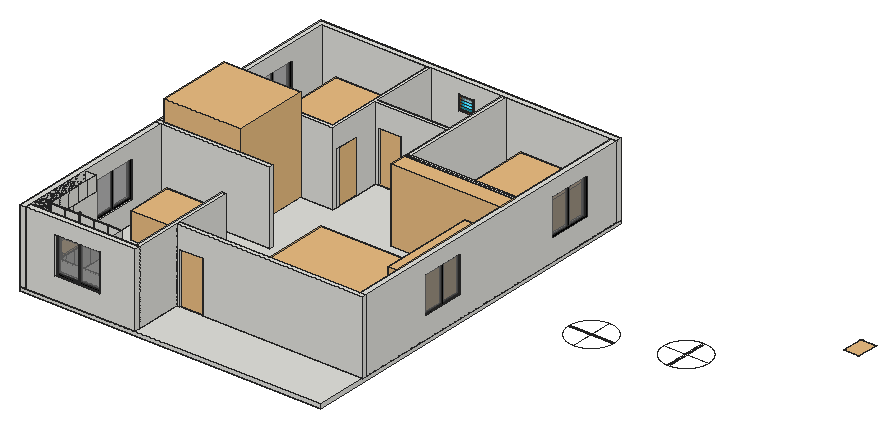
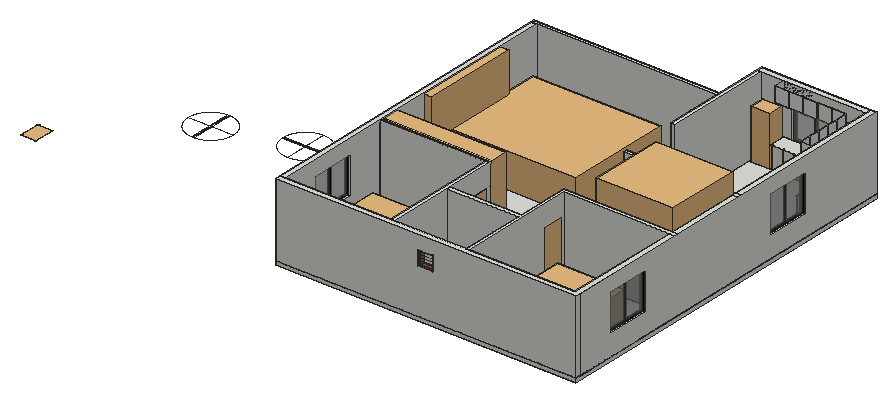
# SketchUp Ruby script. Lengths in inches.
U = 1.inch
M = Sketchup.active_model
def pt(a) = Geom::Point3d.new(a.map { |v| v * U })
def face(e, loops, mat)
  f = e.add_face(loops[0].map { |a| pt(a) })
  loops[1..].each { |l| e.add_face(l.map { |a| pt(a) }).erase! }
  f.material = f.back_material = mat if mat
  f
end
# faces: each face lists its corners as indices into pts; further lists are holes
def faces(e, pts, list, mat = nil) = list.each { |f| face(e, (f[0].is_a?(Array) ? f : [f]).map { |l| l.map { |i| pts[i] } }, mat) }
# xy, xz, yz: faces in a plane at the given z, y or x. An outline is a flat list of corners, or four numbers for a rectangle; further outlines are holes
def ring(l) = l.size == 4 ? [[l[0], l[1]], [l[2], l[1]], [l[2], l[3]], [l[0], l[3]]] : l.each_slice(2).to_a
def flat(e, list, mat, &to3) = list.each { |f| face(e, (f[0].is_a?(Array) ? f : [f]).map { |l| ring(l).map { |u, v| to3.(u, v) } }, mat) }
def xy(e, z, list, mat = nil) = flat(e, list, mat) { |x, y| [x, y, z] }
def xz(e, y, list, mat = nil) = flat(e, list, mat) { |x, z| [x, y, z] }
def yz(e, x, list, mat = nil) = flat(e, list, mat) { |y, z| [x, y, z] }
def lines(e, pts, list) = list.each { |a, b| e.add_line(pt(pts[a]), pt(pts[b])) }
# prism: a flat outline (further loops are holes) pulled along v
def prism(e, loops, v, mat = nil)
  f = face(e, loops, mat); d = Geom::Vector3d.new(v.map { |x| x * U })
  f.pushpull(f.normal.samedirection?(d) ? d.length : -d.length)
end
def box(e, o, s, mat = nil) = prism(e, [[o, [o[0] + s[0], o[1], o[2]], [o[0] + s[0], o[1] + s[1], o[2]], [o[0], o[1] + s[1], o[2]]]], [0, 0, s[2]], mat)
def at(x, y, z, deg = 0) = Geom::Transformation.translation(pt([x, y, z])) * Geom::Transformation.rotation(ORIGIN, Z_AXIS, deg.degrees)
def axes(o, x, y, z) = Geom::Transformation.new([*x, 0, *y, 0, *z, 0, *pt(o).to_a, 1])
def part(name) = M.definitions.add(name)
# library, detail: a bought-in or finely detailed component or shape, given as its bounding box
def library(name, o, s) = part(name).tap { |d| box(d.entities, o, s) }
def detail(e, o, s) = box(e.add_group.entities, o, s)
def put(e, d, t, mat = nil) = e.add_instance(d, t).tap { |i| i.material = mat if mat }
def group(e, t, mat = nil) = e.add_group.tap { |g| g.transformation = t; g.material = mat if mat }.entities
root = M.entities
M.materials.add("[Color_008]").color = [30, 30, 30]
M.materials.add("[Color_009]").color = [0, 0, 0]
M.materials.add("[Translucent Glass Gray]").color = [128, 128, 128]
M.materials["[Translucent Glass Gray]"].alpha = 0.5
M.materials.add("[Translucent Glass Tinted]1").color = [7, 201, 240]
M.materials["[Translucent Glass Tinted]1"].alpha = 0.48
M.materials.add("[Translucent_Glass_Gray]").color = [128, 128, 128]
M.materials["[Translucent_Glass_Gray]"].alpha = 0.5
M.materials.add("[Wood Cherry Original]").color = [152, 86, 42]
M.materials.add("[Wood Floor Parquet]").color = [145, 89, 39]
c1 = library("bed",[-25.65,-58.99,0],[75.48,89.46,37.24])
c2 = library("sofa+(2)",[-100.93,-81.02,-0.06],[174.43,145.32,46.54])
c3 = library("DINING+TABLE_4+SEATER_+1200mm+x+900mm",[14.07,13.24,0],[72.26,62.1,36.02])
c4 = library("main+door",[0,-0.79,0],[47.24,7.88,82.68])
c5 = part("ventilator")
g1 = group(c5.entities,at(0,0,0))
xy(g1,0,[[0,0,24,1],[0,1,24,6.83]],"[Wood Floor Parquet]")
xy(g1,1.75,[[2,0,22,6.83]],"[Wood Floor Parquet]")
xy(g1,21.87,[[2,0,22,6.83]],"[Wood Cherry Original]")
xy(g1,23.62,[[0,0,24,1],[0,1,24,6.83]],"[Wood Floor Parquet]")
xz(g1,0,[[[0,0,24,23.62],[2,1.75,22,21.87]]],"[Wood Floor Parquet]")
xz(g1,6.83,[[[0,0,24,23.62],[2,1.75,22,21.87]]],"[Wood Cherry Original]")
yz(g1,0,[[0,0,1,23.62],[1,0,6.83,23.62]],"[Wood Floor Parquet]")
yz(g1,2,[[0,1.75,6.83,1.75,6.83,7.66,0,3.5],[0,3.5,6.83,7.66,6.83,11.8125,0,7.66],[0,7.66,6.83,11.8125,6.83,15.97,0,11.8125],[0,11.8125,6.83,15.97,6.83,20.12,0,15.97],[0,15.97,6.83,20.12,6.83,21.87,0,21.87]],"[Wood Floor Parquet]")
yz(g1,22,[[0,1.75,0,3.5,6.83,7.66,6.83,1.75],[0,3.5,0,7.66,6.83,11.8125,6.83,7.66],[0,7.66,0,11.8125,6.83,15.97,6.83,11.8125],[0,11.8125,0,15.97,6.83,20.12,6.83,15.97],[0,15.97,0,21.87,6.83,21.87,6.83,20.12]],"[Wood Floor Parquet]")
yz(g1,24,[[0,0,1,23.62],[1,0,6.83,23.62]],"[Wood Floor Parquet]")
p = [[2,0,3.5],[2,6.83,7.66],[22,6.83,7.66],[22,0,3.5],[2,6.83,11.8125],[2,0,7.66],
  [22,0,7.66],[22,6.83,11.8125],[2,0,11.8125],[2,6.83,15.97],[22,6.83,15.97],[22,0,11.8125],
  [2,6.83,20.12],[2,0,15.97],[22,0,15.97],[22,6.83,20.12]]
faces(g1,p,[[0,1,2,3],[4,5,6,7],[8,9,10,11]],"[Translucent Glass Tinted]1")
faces(g1,p,[[12,13,14,15]],"[Translucent Glass Gray]")
c6 = part("Group\#2")
xy(c6.entities,0,[[0,0,82.68,1.18]],"[Color_009]")
xy(c6.entities,1.97,[[1.97,0.98,40.35,1.18],[42.32,0.98,80.71,1.18]])
xy(c6.entities,1.97,[[1.97,0,40.35,0.3],[42.32,0,80.71,0.3]],"[Color_009]")
xy(c6.entities,80.71,[[1.97,0,40.35,0.3],[42.32,0,80.71,0.3],[1.97,0.3,40.35,0.98],[42.32,0.3,80.71,0.98],[1.97,0.98,40.35,1.18],
  [42.32,0.98,80.71,1.18]])
xy(c6.entities,82.68,[[0,0,82.68,1.18]],"[Color_008]")
xz(c6.entities,0,[[[0,0,82.68,82.68],[1.97,1.97,40.35,80.71],[42.32,1.97,80.71,80.71]]],"[Color_009]")
xz(c6.entities,0.3,[[1.97,1.97,40.35,80.71],[42.32,1.97,80.71,80.71]],"[Translucent_Glass_Gray]")
xz(c6.entities,0.98,[[1.97,1.97,40.35,80.71],[42.32,1.97,80.71,80.71]],"[Translucent_Glass_Gray]")
xz(c6.entities,1.18,[[[0,0,82.68,82.68],[1.97,1.97,80.71,80.71]],[40.35,1.97,42.32,80.71]],"[Color_009]")
yz(c6.entities,0,[[0,0,1.18,82.68]],"[Color_009]")
yz(c6.entities,1.97,[[0.98,1.97,1.18,80.71]])
yz(c6.entities,1.97,[[0,1.97,0.3,80.71]],"[Color_009]")
yz(c6.entities,40.35,[[0,1.97,0.3,80.71],[0.98,1.97,1.18,80.71]],"[Color_009]")
yz(c6.entities,42.32,[[0,1.97,0.3,80.71],[0.98,1.97,1.18,80.71]])
yz(c6.entities,80.71,[[0,1.97,0.3,80.71],[0.98,1.97,1.18,80.71]],"[Color_009]")
yz(c6.entities,82.68,[[0,0,1.18,82.68]],"[Color_009]")
c7 = library("A$C150B42AD",[-2.96,-4.03,0],[5.92,8.06,0.01])
c8 = library("Component\#33",[0,0,0],[60.64,55.48,158.625])
c9 = library("CS300DRT",[0,0,0],[27.18,17.85,30.31])
c10 = library("Group\#6",[0,0,0],[122,120,150.6])
c11 = library("Group\#13",[0,-2.07,0],[175.11,29.89,117.3125])
c12 = library("Curtain set",[2.63,-1.46,0.02],[153.32,14.02,114.15])
c13 = library("Gas range top",[0,0,34.52],[24.41,48.07,2.63])
c14 = library("SKT_Nearly Natural 5' Kentia Palm Silk Tree",[-23.18,-17.61,0],[47.48,43.95,59.125])
c15 = part("Inclined chimney")
g2 = group(c15.entities,at(1.97,2.08,2.89))
xy(g2,0,[[0,7.9,31.3,13.68]])
xy(g2,11.29,[[0,0,31.3,13.68]])
xz(g2,13.68,[[0,0,31.3,11.29]])
yz(g2,0,[[7.9,0,0,11.29,13.68,11.29,13.68,0]])
yz(g2,31.3,[[7.9,0,13.68,0,13.68,11.29,0,11.29]])
g3 = group(c15.entities,at(0,9.85,0.4))
g4 = group(g3,at(0,0.61,0.43))
prism(g4,[[[35.24,0,0],[35.24,-3.39,4.84],[35.24,-3.58,4.7],[35.24,-0.29,0]]],[-35.24,0,0])
g5 = group(g3,at(0,-3.21,4.99))
prism(g5,[[[35.24,-0.2,-0.12],[35.24,-3.16,5],[0,-3.16,5],[0,-0.2,-0.12]]],[0,0.2,0.12])
g6 = group(g3,at(0,-6.27,10.27))
prism(g6,[[[35.24,-0.19,-0.14],[35.24,-3.58,4.7],[0,-3.58,4.7],[0,-0.19,-0.14]]],[0,0.19,0.14])
g7 = group(g3,at(0,0.61,0.43))
prism(g7,[[[35.24,0,0],[35.24,0.96,0],[35.24,-9.52,14.96],[35.24,-10.16,14.51]]],[-35.24,0,0])
g8 = group(c15.entities,at(10.24,3.95,20.8))
box(g8,[0,0,-6.62],[14.76,11.8125,20.56])
g9 = group(c15.entities,at(0,10.1,0))
prism(g9,[[[35.24,0.46,0],[35.24,1.33,0],[35.24,1.33,0.83],[35.24,1.01,0.83],[35.24,0.37,0.83],[35.24,0,0.83],[35.24,0,0.64]]],[-35.24,0,0])
c16 = part("Inclined+chimney")
put(c16.entities,c15,at(34.17,38.97,0.69))
xy(root,0,[[259.625,9,283.625,32.9],[259.625,32.9,283.625,104.9]])
xy(root,0.2,[[283.82,32.9,301.42,33.08],[301.82,32.9,319.42,33.08],[319.82,32.9,355.42,33.08],[355.82,32.9,373.42,33.08],[373.82,32.9,391.42,33.08],
  [283.625,33.1,283.8,49.49],[283.625,49.89,283.8,66.28],[283.625,66.68,283.8,80.9],[283.625,80.9,283.8,83.07],[283.625,83.47,283.8,99.85],
  [283.625,100.25,283.8,104.9],[283.625,104.9,283.8,116.64]])
xy(root,11.8,[[319.82,32.9,355.42,33.08]])
xy(root,12.2,[[319.82,32.9,355.42,33.08]])
xy(root,23.8,[[319.82,32.9,355.42,33.08]])
xy(root,24.2,[[319.82,32.9,355.42,33.08]])
xy(root,35.8,[[283.82,32.9,301.42,33.08],[301.82,32.9,319.42,33.08],[319.82,32.9,355.42,33.08],[355.82,32.9,373.42,33.08],[373.82,32.9,391.42,33.08],
  [283.625,33.1,283.8,49.49],[283.625,49.89,283.8,66.28],[283.625,66.68,283.8,83.07],[283.625,83.47,283.8,99.85],[283.625,100.25,283.8,116.64]])
xy(root,93.9375,[[259.625,9,277.625,116.84],[277.625,9,391.625,27]])
xy(root,94.14,[[277.82,27,300.22,27.18],[300.625,27,323.02,27.18],[323.42,27,345.82,27.18],[346.22,27,368.625,27.18],[369.02,27,391.42,27.18],
  [277.625,27.2,277.8,44.77],[277.625,45.17,277.8,62.74],[277.625,63.14,277.8,80.71],[277.625,81.11,277.8,98.67],[277.625,99.07,277.8,116.64]])
xz(root,9,[[259.625,93.9375,391.625,117.3125]])
xz(root,27,[[[277.625,93.9375,300.42,117.3125],[277.82,94.14,300.22,117.11]],[[300.42,93.9375,323.22,117.3125],[300.625,94.14,323.02,117.11]],[[323.22,93.9375,346.02,117.3125],[323.42,94.14,345.82,117.11]],[[346.02,93.9375,368.82,117.3125],[346.22,94.14,368.625,117.11]],[[368.82,93.9375,391.625,117.3125],[369.02,94.14,391.42,117.11]]])
xz(root,27.18,[[277.82,94.14,300.22,117.11],[300.625,94.14,323.02,117.11],[323.42,94.14,345.82,117.11],[346.22,94.14,368.625,117.11],[369.02,94.14,391.42,117.11]])
xz(root,27.2,[[277.625,94.14,277.8,117.11]])
xz(root,32.9,[[[283.625,0,301.625,36],[283.82,0.2,301.42,35.8]],[[301.625,0,319.625,36],[301.82,0.2,319.42,35.8]],[[319.625,0,355.625,12],[319.82,0.2,355.42,11.8]],[[355.625,0,373.625,36],[355.82,0.2,373.42,35.8]],[[373.625,0,391.625,36],[373.82,0.2,391.42,35.8]],
  [[319.625,12,355.625,24],[319.82,12.2,355.42,23.8]],[[319.625,24,355.625,36],[319.82,24.2,355.42,35.8]]])
xz(root,33.08,[[283.82,0.2,301.42,35.8],[301.82,0.2,319.42,35.8],[319.82,0.2,355.42,11.8],[355.82,0.2,373.42,35.8],[373.82,0.2,391.42,35.8],
  [319.82,12.2,355.42,23.8],[319.82,24.2,355.42,35.8]])
xz(root,33.1,[[283.625,0.2,283.8,35.8]])
xz(root,44.77,[[277.625,94.14,277.8,117.11]])
xz(root,45.17,[[277.625,94.14,277.8,117.11]])
xz(root,49.49,[[283.625,0.2,283.8,35.8]])
xz(root,49.89,[[283.625,0.2,283.8,35.8]])
xz(root,62.74,[[277.625,94.14,277.8,117.11]])
xz(root,63.14,[[277.625,94.14,277.8,117.11]])
xz(root,66.28,[[283.625,0.2,283.8,35.8]])
xz(root,66.68,[[283.625,0.2,283.8,35.8]])
xz(root,80.71,[[277.625,94.14,277.8,117.11]])
xz(root,81.11,[[277.625,94.14,277.8,117.11]])
xz(root,83.07,[[283.625,0.2,283.8,35.8]])
xz(root,83.47,[[283.625,0.2,283.8,35.8]])
xz(root,98.67,[[277.625,94.14,277.8,117.11]])
xz(root,99.07,[[277.625,94.14,277.8,117.11]])
xz(root,99.85,[[283.625,0.2,283.8,35.8]])
xz(root,100.25,[[283.625,0.2,283.8,35.8]])
xz(root,116.64,[[283.625,0.2,283.8,35.8],[277.625,94.14,277.8,117.11]])
xz(root,116.84,[[259.625,93.9375,277.625,117.3125]])
yz(root,259.625,[[9,93.9375,116.84,117.3125]])
yz(root,277.625,[[[27,93.9375,44.97,117.3125],[27.2,94.14,44.77,117.11]],[[44.97,93.9375,62.9375,117.3125],[45.17,94.14,62.74,117.11]],[[62.9375,93.9375,80.91,117.3125],[63.14,94.14,80.71,117.11]],[[80.91,93.9375,98.875,117.3125],[81.11,94.14,98.67,117.11]],[[98.875,93.9375,116.84,117.3125],[99.07,94.14,116.64,117.11]]])
yz(root,277.8,[[27.2,94.14,44.77,117.11],[45.17,94.14,62.74,117.11],[63.14,94.14,80.71,117.11],[81.11,94.14,98.67,117.11],[99.07,94.14,116.64,117.11]])
yz(root,277.82,[[27,94.14,27.18,117.11]])
yz(root,283.625,[[[32.9,0,116.84,36],[66.68,0.2,83.07,35.8],[49.89,0.2,66.28,35.8],[33.1,0.2,49.49,35.8],[83.47,0.2,99.85,35.8],[100.25,0.2,116.64,35.8]]])
yz(root,283.8,[[33.1,0.2,49.49,35.8],[49.89,0.2,66.28,35.8],[66.68,0.2,83.07,35.8],[83.47,0.2,99.85,35.8],[100.25,0.2,116.64,35.8]])
yz(root,283.82,[[32.9,0.2,33.08,35.8]])
yz(root,300.22,[[27,94.14,27.18,117.11]])
yz(root,300.625,[[27,94.14,27.18,117.11]])
yz(root,301.42,[[32.9,0.2,33.08,35.8]])
yz(root,301.82,[[32.9,0.2,33.08,35.8]])
yz(root,319.42,[[32.9,0.2,33.08,12],[32.9,12,33.08,24],[32.9,24,33.08,35.8]])
yz(root,319.82,[[32.9,0.2,33.08,11.8],[32.9,12.2,33.08,23.8],[32.9,24.2,33.08,35.8]])
yz(root,323.02,[[27,94.14,27.18,117.11]])
yz(root,323.42,[[27,94.14,27.18,117.11]])
yz(root,345.82,[[27,94.14,27.18,117.11]])
yz(root,346.22,[[27,94.14,27.18,117.11]])
yz(root,355.42,[[32.9,0.2,33.08,11.8],[32.9,12.2,33.08,23.8],[32.9,24.2,33.08,35.8]])
yz(root,355.82,[[32.9,0.2,33.08,12],[32.9,12,33.08,24],[32.9,24,33.08,35.8]])
yz(root,368.625,[[27,94.14,27.18,117.11]])
yz(root,369.02,[[27,94.14,27.18,117.11]])
yz(root,373.42,[[32.9,0.2,33.08,35.8]])
yz(root,373.82,[[32.9,0.2,33.08,35.8]])
yz(root,391.42,[[32.9,0.2,33.08,35.8],[27,94.14,27.18,117.11]])
yz(root,391.625,[[9,93.9375,27,117.3125]])
p = [[1002.83,347.84,0],[1005.08,347.63,0],[971.98,390.31,0],[971.63,388.07,0],[973.87,396.8125,0],[973.11,394.69,0],
  [1000.6,348.2,0],[972.47,392.51,0],[984.4,411.3,0],[982.7,409.8,0],[996.22,417.8,0],[994.09,417.03,0],
  [981.1,408.2,0],[979.61,406.51,0],[992.02,416.13,0],[990,415.11,0],[978.22,404.72,0],[976.95,402.85,0],
  [971.41,385.82,0],[971.34,383.5625,0],[1005.34,347.625,0],[975.8,400.9,0],[1005.08,419.49,0],[1002.83,419.28,0],
  [1000.6,418.92,0],[998.39,418.43,0],[974.77,398.89,0],[986.18,412.69,0],[988.05,413.96,0],[1035.08,360.61,0],
  [1036.47,362.4,0],[876.33,314.25,0],[878.57,313.9,0],[1024.6875,352.01,0],[1026.63,353.16,0],[1009.34,347.5625,0],
  [1009.34,347.625,0],[865.73,318.07,0],[867.75,317.04,0],[880.82,313.6875,0],[1007.34,347.5625,0],[1018.47,349.32,0],
  [1020.6,350.09,0],[1033.59,358.92,0],[1016.3,348.69,0],[871.95,315.38,0],[874.125,314.75,0],[1007.34,383.5625,0],
  [1009.34,383.5625,0],[1037.74,364.27,0],[1038.89,366.22,0],[1039.92,368.23,0],[1040.82,370.31,0],[1041.58,372.4375,0],
  [1007.34,419.5625,0],[1022.67,350.99,0],[869.83,316.14,0],[1011.86,347.84,0],[1014.09,348.2,0],[1009.6,347.63,0],
  [1030.29,355.82,0],[1031.99,357.32,0],[1028.5,354.4375,0],[1042.21,374.61,0],[883.08,313.62,0],[1042.71,376.81,0],
  [1043.06,379.05,0],[1043.27,381.3,0],[1043.34,383.5625,0],[860.13,377.35,0],[858.43,375.86,0],[853.95,370.78,0],
  [852.68,368.91,0],[883.08,349.62,0],[883.08,347.62,0],[867.75,382.19,0],[865.73,381.16,0],[861.92,378.74,0],
  [856.83,374.26,0],[855.34,372.5625,0],[850.5,364.94,0],[849.61,362.87,0],[863.79,380.01,0],[847.72,356.36,0],
  [847.36,354.13,0],[847.15,351.875,0],[851.53,366.96,0],[848.84,360.74,0],[847.14,351.62,0],[848.21,358.57,0],
  [919.08,349.62,0],[919.08,347.62,0],[919.01,347.62,0],[887.59,313.9,0],[889.82,314.25,0],[913.47,330.33,0],
  [914.625,332.27,0],[885.34,313.6875,0],[907.72,323.375,0],[909.32,324.97,0],[915.65,334.29,0],[916.55,336.36,0],
  [917.32,338.49,0],[917.95,340.66,0],[898.41,317.04,0],[900.42,318.07,0],[894.2,315.38,0],[896.33,316.14,0],
  [902.37,319.22,0],[904.24,320.49,0],[892.03,314.75,0],[906.03,321.88,0],[910.82,326.67,0],[912.2,328.46,0],
  [918.44,342.87,0],[855.34,326.67,0],[856.83,324.97,0],[847.08,349.62,0],[847.08,347.62,0],[860.13,321.88,0],
  [861.92,320.49,0],[863.79,319.22,0],[847.14,347.62,0],[848.21,340.66,0],[848.84,338.49,0],[851.53,332.27,0],
  [852.68,330.33,0],[858.43,323.375,0],[847.72,342.87,0],[853.95,328.46,0],[918.79,345.1,0],[847.15,347.36,0],
  [847.36,345.1,0],[849.61,336.36,0],[850.5,334.29,0],[919.01,347.36,0],[971.41,381.3,0],[1005.34,347.5625,0],
  [971.63,379.05,0],[971.98,376.81,0],[972.47,374.61,0],[973.11,372.4375,0],[973.87,370.31,0],[974.77,368.23,0],
  [975.8,366.22,0],[976.95,364.27,0],[978.22,362.4,0],[982.7,357.32,0],[984.4,355.82,0],[979.61,360.61,0],
  [981.1,358.92,0],[988.05,353.16,0],[990,352.01,0],[992.02,350.99,0],[1005.34,383.5625,0],[986.18,354.4375,0],
  [994.09,350.09,0],[996.22,349.32,0],[998.39,348.69,0],[910.82,372.5625,0],[909.32,374.26,0],[907.72,375.86,0],
  [919.01,351.875,0],[918.79,354.13,0],[918.44,356.36,0],[917.95,358.57,0],[917.32,360.74,0],[919.08,351.62,0],
  [919.01,351.62,0],[916.55,362.87,0],[915.65,364.94,0],[914.625,366.96,0],[913.47,368.91,0],[912.2,370.78,0],
  [883.08,351.62,0],[874.125,384.49,0],[871.95,383.85,0],[889.82,384.98,0],[887.59,385.33,0],[869.83,383.09,0],
  [906.03,377.35,0],[880.82,385.55,0],[878.57,385.33,0],[885.34,385.55,0],[902.37,380.01,0],[900.42,381.16,0],
  [894.2,383.85,0],[892.03,384.49,0],[876.33,384.98,0],[896.33,383.09,0],[847.08,351.62,0],[898.41,382.19,0],
  [904.24,378.74,0],[883.08,385.62,0],[1005.34,419.5,0],[1009.34,419.5,0],[1005.34,419.5625,0],[1043.27,385.82,0],
  [1009.34,419.5625,0],[1043.06,388.07,0],[1042.71,390.31,0],[1042.21,392.51,0],[1041.58,394.69,0],[1037.74,402.85,0],
  [1036.47,404.72,0],[1035.08,406.51,0],[1033.59,408.2,0],[1031.99,409.8,0],[1026.63,413.96,0],[1024.6875,415.11,0],
  [1014.09,418.92,0],[1011.86,419.28,0],[1040.82,396.8125,0],[1039.92,398.89,0],[1030.29,411.3,0],[1028.5,412.69,0],
  [1022.67,416.13,0],[1020.6,417.03,0],[1038.89,400.9,0],[1018.47,417.8,0],[1016.3,418.43,0],[1009.6,419.49,0],
  [259.625,402,0],[250.625,402,0],[250.625,460.5,0],[255.125,460.5,0],[726.125,280.5,0],[726.125,244.5,0],
  [721.625,496.5,0],[726.125,496.5,0],[430.625,486,0],[433.625,486,0],[351.625,354,0],[351.625,396,0],
  [474.625,480,0],[547.625,480,0],[427.625,591,0],[427.625,443,0],[250.625,177,0],[255.125,177,0],
  [433.625,407,0],[433.625,402,0],[250.625,496.5,0],[255.125,496.5,0],[721.625,532.5,0],[726.125,532.5,0],
  [331.625,354,0],[331.625,396,0],[381.625,396,0],[371.625,396,0],[427.625,402,0],[381.625,354,0],
  [371.625,354,0],[726.125,460.5,0],[361.625,354,0],[361.625,396,0],[427.625,600,0],[250.625,532.5,0],
  [255.125,532.5,0],[721.625,244.5,0],[721.625,402,0],[553.625,402,0],[427.625,276,0],[427.625,270,0],
  [341.625,354,0],[341.625,396,0],[730.625,402,0],[553.625,443,0],[553.625,591,0],[250.625,213,0],
  [255.125,213,0],[721.625,280.5,0],[547.625,443,0],[427.625,396,0],[474.625,486,0],[547.625,486,0],
  [433.625,396,0],[721.625,208.5,0],[726.125,208.5,0],[721.625,84,0],[721.625,90,0],[721.625,460.5,0],
  [250.625,141,0],[255.125,141,0],[433.625,443,0],[433.625,600,0],[433.625,591,0],[259.625,591,0],
  [250.625,591,0],[490.625,591,0],[490.625,595.5,0],[502.625,591,0],[502.625,595.5,0],[478.625,591,0],
  [721.625,600,0],[553.625,600,0],[547.625,591,0],[730.625,460.5,0],[478.625,595.5,0],[321.625,276,0],
  [311.625,276,0],[427.625,0,0],[433.625,0,0],[433.625,84,0],[474.625,84,0],[301.625,276,0],
  [730.625,396,0],[721.625,396,0],[730.625,84,0],[730.625,90,0],[259.625,600,0],[433.625,270,0],
  [553.625,396,0],[730.625,496.5,0],[730.625,532.5,0],[433.625,276,0],[321.625,396,0],[311.625,396,0],
  [430.625,480,0],[433.625,480,0],[547.625,396,0],[547.625,402,0],[474.625,90,0],[721.625,591,0],
  [259.625,0,0],[306.125,0,0],[331.625,276,0],[583.625,409,0],[583.5625,409,0],[547.625,407,0],
  [553.625,407,0],[440.625,516,0],[440.625,515.9375,0],[427.625,407,0],[397.625,409,0],[397.6875,409,0],
  [721.625,93,0],[433.625,181.5,0],[427.625,181.5,0],[438.625,480,0],[730.625,591,0],[730.625,600,0],
  [547.625,600,0],[427.625,32.9,0],[259.625,318,0],[259.625,276,0],[250.625,318,0],[259.625,354,0],
  [381.625,318,0],[381.625,276,0],[259.625,270,0],[730.625,208.5,0],[490.625,600,0],[502.625,600,0],
  [259.625,396,0],[478.625,600,0],[730.625,244.5,0],[259.625,460.5,0],[550.625,600,0],[351.625,276,0],
  [341.625,276,0],[378.125,0,0],[301.625,354,0],[250.625,9,0],[250.625,0,0],[250.625,354,0],
  [301.625,396,0],[250.625,396,0],[378.125,4.5,0],[433.625,9,0],[259.625,9,0],[429.76,32.9,0],
  [250.625,600,0],[427.625,9,0],[301.625,318,0],[250.625,276,0],[311.625,318,0],[311.625,354,0],
  [331.625,318,0],[321.625,318,0],[342.125,0,0],[321.625,354,0],[341.625,318,0],[351.625,318,0],
  [259.625,213,0],[430.625,600,0],[730.625,280.5,0],[250.625,270,0],[342.125,4.5,0],[438.625,486,0],
  [259.625,496.5,0],[361.625,318,0],[259.625,532.5,0],[306.125,4.5,0],[306.125,9,0],[342.125,9,0],
  [378.125,9,0],[259.625,141,0],[259.625,177,0],[550.625,480,0],[550.625,486,0],[259.625,104.9,0],
  [283.625,9,0],[259.625,9,36],[259.625,9,93.9375],[391.625,32.9,0],[361.625,276,0],[371.625,276,0],
  [371.625,318,0]]
lines(root,p,[[0,1],[2,3],[4,5],[6,0],[7,2],[8,9],[10,11],[9,12],[12,13],[11,14],[14,15],[16,17],
  [5,7],[18,19],[1,20],[17,21],[22,23],[23,24],[24,25],[26,4],[25,10],[27,8],[13,16],[28,27],
  [21,26],[3,18],[15,28],[29,30],[31,32],[33,34],[35,36],[37,38],[32,39],[40,36],[41,42],[43,29],
  [44,41],[45,46],[47,48],[49,50],[50,51],[52,53],[47,54],[46,31],[42,55],[38,56],[30,49],[57,58],
  [59,57],[60,61],[61,43],[55,33],[34,62],[56,45],[62,60],[53,63],[39,64],[40,35],[63,65],[51,52],
  [65,66],[66,67],[67,68],[47,40],[58,44],[69,70],[71,72],[73,74],[75,76],[77,69],[70,78],[79,71],
  [78,79],[80,81],[82,77],[83,84],[84,85],[86,80],[81,87],[85,88],[76,82],[89,83],[90,91],[91,92],
  [87,89],[72,86],[93,94],[95,96],[64,97],[98,99],[100,101],[102,103],[104,105],[106,107],[108,109],[97,93],
  [110,106],[111,98],[105,108],[99,112],[94,110],[112,113],[113,95],[107,104],[109,111],[96,100],[101,102],[103,114],
  [115,116],[117,118],[119,120],[121,37],[118,122],[123,124],[125,126],[116,127],[127,119],[120,121],[128,123],[126,129],
  [114,130],[131,132],[132,128],[124,133],[117,122],[133,134],[134,125],[130,135],[135,92],[129,115],[19,136],[40,137],
  [136,138],[138,139],[139,140],[141,142],[137,20],[143,144],[144,145],[145,146],[147,148],[149,150],[151,152],[152,153],
  [140,141],[146,149],[47,154],[142,143],[150,147],[148,155],[155,151],[153,156],[157,158],[158,6],[156,157],[159,160],
  [160,161],[162,163],[164,165],[165,166],[163,164],[73,90],[167,168],[166,169],[170,171],[169,170],[90,168],[172,173],
  [73,174],[173,159],[171,172],[90,167],[175,176],[177,178],[176,179],[161,180],[179,75],[181,182],[178,183],[184,185],
  [73,117],[186,187],[182,188],[189,186],[190,88],[191,189],[180,192],[187,177],[117,190],[183,193],[193,181],[185,191],
  [188,175],[192,184],[194,22],[20,40],[194,154],[36,48],[36,59],[48,68],[195,48],[74,64],[88,117],[92,74],
  [122,74],[122,131],[92,90],[20,154],[154,19],[168,174],[168,162],[174,193],[88,174],[54,194],[54,196],[196,194],
  [68,197],[54,198],[198,195],[197,199],[199,200],[200,201],[201,202],[195,54],[203,204],[205,206],[204,205],[206,207],
  [208,209],[210,211],[212,213],[214,215],[215,208],[216,217],[213,218],[218,203],[207,214],[217,219],[219,220],[202,212],
  [211,221],[220,210],[221,195],[209,216],[222,223],[224,225],[226,227],[228,229],[230,231],[232,233],[234,235],[236,237],
  [238,239],[240,241],[242,243],[244,245],[246,247],[248,249],[241,250],[251,252],[229,253],[254,255],[256,236],[257,258],
  [252,249],[259,227],[260,261],[262,263],[264,265],[258,243],[266,260],[267,268],[269,270],[271,226],[270,239],[272,235],
  [273,248],[274,275],[274,234],[245,229],[276,273],[277,278],[279,280],[281,253],[282,283],[237,284],[285,286],[286,236],
  [287,288],[289,290],[291,292],[286,293],[294,295],[268,296],[266,297],[298,290],[299,300],[301,302],[236,287],[303,304],
  [300,305],[306,307],[308,309],[310,287],[311,263],[233,265],[312,261],[313,314],[243,225],[228,244],[315,262],[316,317],
  [318,319],[288,257],[320,321],[293,298],[322,304],[315,311],[323,268],[322,280],[281,228],[324,325],[326,299],[327,328],
  [329,330],[229,313],[331,332],[240,333],[334,335],[240,284],[280,336],[337,338],[336,277],[261,321],[339,234],[312,320],
  [293,289],[340,341],[296,342],[338,343],[286,231],[337,303],[344,345],[344,346],[344,347],[348,251],[262,349],[329,272],
  [263,350],[261,330],[289,291],[309,351],[352,353],[290,292],[222,354],[298,355],[319,339],[351,356],[264,246],[357,222],
  [295,358],[359,360],[361,301],[362,347],[363,364],[269,238],[347,365],[282,363],[305,345],[362,366],[354,367],[368,361],
  [291,296],[303,369],[365,346],[370,324],[343,371],[231,319],[341,294],[372,288],[340,323],[364,324],[363,370],[369,302],
  [251,248],[343,373],[307,312],[374,362],[292,353],[290,352],[280,309],[345,375],[310,372],[256,310],[373,301],[300,376],
  [366,354],[232,264],[377,317],[326,378],[355,285],[299,379],[380,361],[342,358],[250,222],[223,367],[381,316],[360,382],
  [260,281],[359,383],[305,374],[307,260],[319,284],[242,224],[384,350],[367,365],[323,294],[385,256],[346,375],[386,306],
  [356,386],[265,247],[325,380],[277,259],[246,381],[347,354],[375,387],[271,307],[353,342],[257,242],[224,223],[285,385],
  [388,368],[339,389],[352,355],[249,255],[255,233],[345,350],[374,344],[254,232],[373,369],[378,379],[377,362],[379,376],
  [390,357],[252,254],[321,329],[381,377],[238,282],[391,383],[392,390],[350,387],[376,374],[383,382],[360,326],[287,392],
  [317,366],[382,378],[272,267],[393,388],[394,393],[333,250],[395,388],[396,368],[304,279],[306,266],[397,398],[235,399],
  [275,400],[398,384],[245,314],[239,283],[268,295],[250,273],[278,351],[227,278],[244,323],[279,308],[388,380],[235,275],
  [243,390],[393,325],[226,386],[241,276],[253,297],[314,340],[247,316],[387,269],[239,398],[270,384],[231,389],[225,357],
  [275,296],[283,397],[258,392],[297,313],[259,271],[227,356],[401,397],[396,373],[395,396],[402,394],[394,395],[403,404],
  [405,343],[406,359],[349,348],[407,406],[348,408],[407,408],[349,407],[408,391],[406,391]])
g10 = group(root,at(250.625,0,-6))
xy(g10,0,[[0,0,480,600]])
xy(g10,6,[[[0,0,480,600],[9,9,9,116.84,33,116.84,33,32.9,141,32.9,141,9]]])
xy(g10,42,[[33,32.9,35,116.84],[35,32.9,141,34.9]])
xy(g10,43,[[9,9,141,9,141,34.9,35,34.9,35,116.84,9,116.84]])
xz(g10,0,[[0,0,480,6]])
xz(g10,9,[[9,6,141,43]])
xz(g10,32.9,[[33,6,141,42]])
xz(g10,34.9,[[35,42,141,43]])
xz(g10,116.84,[[9,6,9,43,35,43,35,42,33,42,33,6]])
xz(g10,600,[[0,0,480,6]])
yz(g10,0,[[0,0,600,6]])
yz(g10,9,[[9,6,116.84,43]])
yz(g10,33,[[32.9,6,116.84,42]])
yz(g10,35,[[34.9,42,116.84,43]])
yz(g10,141,[[9,6,32.9,6,32.9,42,34.9,42,34.9,43,9,43]])
yz(g10,480,[[0,0,600,6]])
put(root,c1,axes([617.21,543.15,-3.12],[1.43,0,0],[0,1.43,0],[0,0,1.43]))
put(root,c1,axes([321.28,543.86,0],[1.43,0,0],[0,1.43,0],[0,0,1.43]))
put(root,c2,axes([594.47,183.76,0.07],[-1.17,0,0],[0,-1.17,0],[0,0,1.17]))
put(root,c3,axes([267.78,162.56,0],[1.17,0,0],[0,1.17,0],[0,0,1.17]))
g11 = group(root,at(250.625,0,0))
xy(g11,0,[[0,0,9,141],[9,0,55.5,9],[55.5,0,183,9],[177,9,183,181.5],[183,84,188,90],
  [224,84,480,90],[471,90,480,208.5],[0,141,9,270],[471,208.5,480,460.5],[297,396,471,402],
  [0,402,9,460.5],[297,402,303,407],[177,443,183,591],[297,443,303,591],[0,460.5,9,591],
  [471,460.5,480,591],[183,480,188,486],[224,480,297,486],[0,591,228,600],[228,591,480,600]])
xy(g11,33.9375,[[55.5,0,127.5,9],[0,141,9,213],[471,208.5,480,280.5],[0,460.5,9,532.5],[471,460.5,480,532.5]])
xy(g11,72,[[228,591,252,600]])
xy(g11,81.75,[[188,480,224,486]])
xy(g11,81.9375,[[188,84,224,90]])
xy(g11,84,[[177,407,183,443],[297,407,303,443]])
xy(g11,93.9375,[[55.5,0,127.5,9],[0,141,9,213],[471,208.5,480,280.5],[0,460.5,9,532.5],[471,460.5,480,532.5]])
xy(g11,96,[[228,591,252,600]])
xy(g11,117.3125,[[0,0,9,270],[9,0,183,9],[177,9,183,181.5],[183,84,480,90],[471,90,480,591],
  [0,270,183,276],[0,276,9,396],[0,396,183,396,183,480,297,480,297,486,183,486,183,591,177,591,177,402,0,402],[297,396,471,402],[0,402,9,402,9,591,480,591,480,600,0,600],
  [297,402,303,591]])
xz(g11,0,[[0,0,9,117.3125],[[9,0,183,117.3125],[55.5,33.9375,127.5,93.9375]]])
xz(g11,9,[[[9,0,177,117.3125],[55.5,33.9375,127.5,93.9375]],[177,0,183,117.3125]])
xz(g11,84,[[183,0,188,0,188,81.9375,224,81.9375,224,0,480,0,480,117.3125,183,117.3125]])
xz(g11,90,[[183,0,183,117.3125,471,117.3125,471,0,224,0,224,81.9375,188,81.9375,188,0],[471,0,480,117.3125]])
xz(g11,141,[[0,33.9375,9,93.9375]])
xz(g11,181.5,[[177,0,183,117.3125]])
xz(g11,208.5,[[471,33.9375,480,93.9375]])
xz(g11,213,[[0,33.9375,9,93.9375]])
xz(g11,270,[[9,0,183,117.3125]])
xz(g11,276,[[9,0,183,117.3125]])
xz(g11,280.5,[[471,33.9375,480,93.9375]])
xz(g11,396,[[9,0,183,117.3125],[297,0,471,117.3125]])
xz(g11,402,[[9,0,177,117.3125],[303,0,471,117.3125]])
xz(g11,407,[[177,0,183,84],[297,0,303,84]])
xz(g11,443,[[177,0,183,84],[297,0,303,84]])
xz(g11,460.5,[[0,33.9375,9,93.9375],[471,33.9375,480,93.9375]])
xz(g11,480,[[183,0,188,0,188,81.75,224,81.75,224,0,297,0,297,117.3125,183,117.3125]])
xz(g11,486,[[183,0,183,117.3125,297,117.3125,297,0,224,0,224,81.75,188,81.75,188,0]])
xz(g11,532.5,[[0,33.9375,9,93.9375],[471,33.9375,480,93.9375]])
xz(g11,591,[[9,0,177,117.3125],[177,0,183,117.3125],[[183,0,297,117.3125],[228,72,252,96]],[297,0,303,117.3125],[303,0,471,117.3125],
  [471,0,480,117.3125]])
xz(g11,600,[[[0,0,480,117.3125],[228,72,252,96]]])
yz(g11,0,[[[0,0,591,117.3125],[460.5,33.9375,532.5,93.9375],[141,33.9375,213,93.9375]],[591,0,600,117.3125]])
yz(g11,9,[[0,0,9,117.3125],[[9,0,270,117.3125],[141,33.9375,213,93.9375]],[276,0,396,117.3125],[[402,0,591,117.3125],[460.5,33.9375,532.5,93.9375]]])
yz(g11,55.5,[[0,33.9375,9,93.9375]])
yz(g11,127.5,[[0,33.9375,9,93.9375]])
yz(g11,177,[[9,0,181.5,117.3125],[402,0,402,117.3125,591,117.3125,591,0,443,0,443,84,407,84,407,0]])
yz(g11,183,[[0,0,9,117.3125],[9,0,84,117.3125],[84,0,90,117.3125],[90,0,181.5,117.3125],[270,0,276,117.3125],
  [396,0,402,0,402,84,443,84,443,0,480,0,480,117.3125,396,117.3125],[402,0,407,84],[486,0,591,117.3125]])
yz(g11,188,[[84,0,90,81.9375],[480,0,486,81.75]])
yz(g11,224,[[84,0,90,81.9375],[480,0,486,81.75]])
yz(g11,228,[[591,72,600,96]])
yz(g11,252,[[591,72,600,96]])
yz(g11,297,[[396,0,396,117.3125,480,117.3125,480,0,443,0,443,84,407,84,407,0],[480,0,486,117.3125],[486,0,591,117.3125]])
yz(g11,303,[[402,0,407,0,407,84,443,84,443,0,591,0,591,117.3125,402,117.3125]])
yz(g11,471,[[[90,0,396,117.3125],[208.5,33.9375,280.5,93.9375]],[396,0,402,117.3125],[[402,0,591,117.3125],[460.5,33.9375,532.5,93.9375]]])
yz(g11,480,[[84,0,90,117.3125],[[90,0,591,117.3125],[208.5,33.9375,280.5,93.9375],[460.5,33.9375,532.5,93.9375]],[591,0,600,117.3125]])
p = [[183,402,84],[177,402,84],[303,402,84],[297,402,84],[33,104.9,0],[33,80.9,0],
  [9,104.9,0]]
lines(g11,p,[[0,1],[2,3],[4,5],[6,4]])
put(g11,c4,axes([186.13,86.54,0],[0.8,0,0],[0,0.36,0],[0,0,0.9798]))
put(g11,c5,axes([228,591,72],[1,0,0],[0,1,0],[0,0,1.016]))
put(g11,c4,axes([178.49,442.72,0],[0,-0.8,0],[0.36,0,0],[0,0,1.016]))
put(g11,c4,axes([297.84,442.82,0],[0,-0.8,0],[0.36,0,0],[0,0,0.9798]))
put(g11,c6,axes([2.95,532.5,33.9375],[0,-0.87086,0],[2.5,0,0],[0,0,0.72571]))
put(g11,c6,axes([2.95,213,33.9375],[0,-0.87086,0],[2.5,0,0],[0,0,0.72571]))
put(g11,c6,axes([475.5,280.5,33.9375],[0,-0.87086,0],[2.5,0,0],[0,0,0.72571]))
put(g11,c6,axes([475.5,532.5,33.9375],[0,-0.87086,0],[2.5,0,0],[0,0,0.72571]))
put(g11,c6,axes([55.5,4.5,33.9375],[0.87086,0,0],[0,2.5,0],[0,0,0.72571]))
put(root,c7,axes([1166.18,532.05,0],[4.26064,0,0],[0,4.26064,0],[0,0,4.26064]))
put(root,c8,axes([424.49,32.9,0],[-0.5,0,0],[0,-0.5,0],[0,0,0.5]))
put(root,c9,axes([474.5,591,0],[0,-1.65,0],[1.65,0,0],[0,0,1.65]))
put(root,c7,axes([490.28,570.1875,0],[4.26064,0,0],[0,4.26064,0],[0,0,4.26064]))
put(root,c10,at(259.625,276,0))
put(root,c4,axes([436.76,482.54,0],[0.8,0,0],[0,0.36,0],[0,0,0.9798]))
put(root,c11,at(547.6,370.3,0))
put(root,c12,at(709.07,318.15,3.14,-90))
put(root,c13,at(261.21,44.23,2.48))
put(root,c14,axes([273.85,19.21,37],[0.59,0,0],[0,0.59,0],[0,0,0.59]))
put(root,c16,at(314.36,19.5625,59.34,90))
